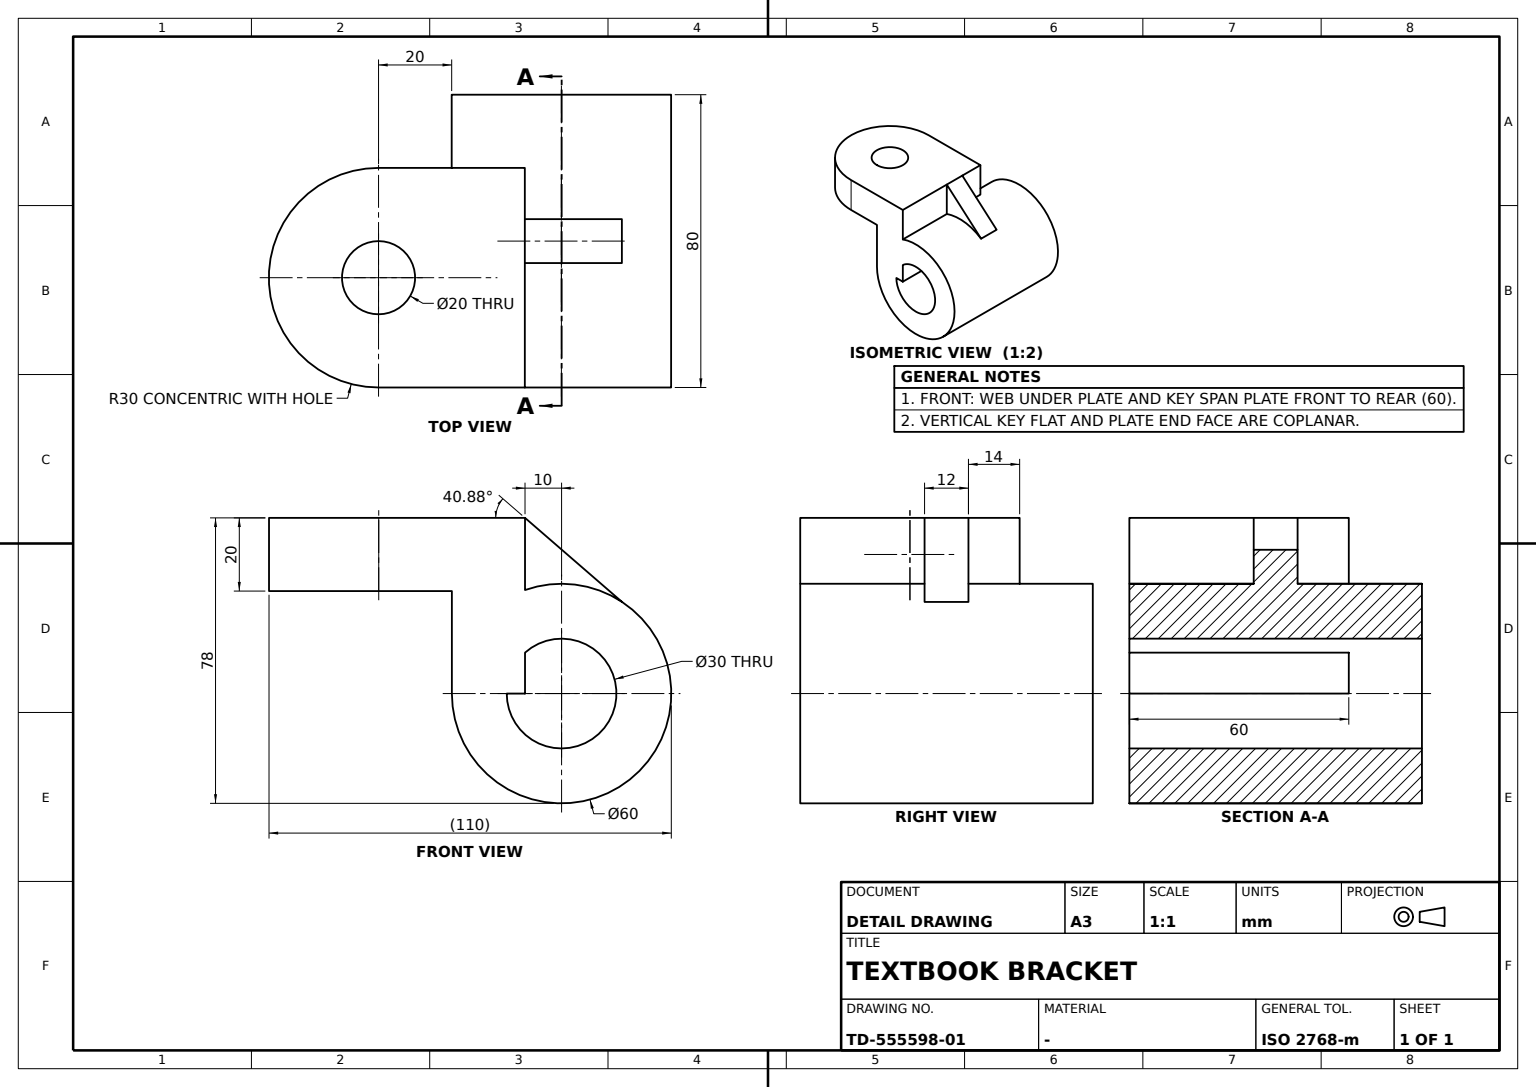
ISO-10303-21;
HEADER;
FILE_DESCRIPTION((''),'2;1');
FILE_NAME('','',(''),(''),'','','');
FILE_SCHEMA(('AUTOMOTIVE_DESIGN'));
ENDSEC;
DATA;
#1=APPLICATION_CONTEXT('');
#2=PRODUCT_CONTEXT('',#1,'mechanical');
#3=PRODUCT('','','',(#2));
#4=PRODUCT_DEFINITION_FORMATION('','',#3);
#5=PRODUCT_DEFINITION_CONTEXT('',#1,'design');
#6=PRODUCT_DEFINITION('','',#4,#5);
#7=PRODUCT_DEFINITION_SHAPE('','',#6);
#8=(LENGTH_UNIT()NAMED_UNIT(*)SI_UNIT(.MILLI.,.METRE.));
#9=(NAMED_UNIT(*)PLANE_ANGLE_UNIT()SI_UNIT($,.RADIAN.));
#10=(NAMED_UNIT(*)SI_UNIT($,.STERADIAN.)SOLID_ANGLE_UNIT());
#11=UNCERTAINTY_MEASURE_WITH_UNIT(LENGTH_MEASURE(0.005),#8,'distance_accuracy_value','');
#12=(GEOMETRIC_REPRESENTATION_CONTEXT(3)GLOBAL_UNCERTAINTY_ASSIGNED_CONTEXT((#11))GLOBAL_UNIT_ASSIGNED_CONTEXT((#8,#9,#10))REPRESENTATION_CONTEXT('',''));
#13=CARTESIAN_POINT('',(-34.,10.,48.));
#14=VERTEX_POINT('',#13);
#15=CARTESIAN_POINT('',(-34.,36.536894,25.030604));
#16=VERTEX_POINT('',#15);
#17=DIRECTION('',(0.,0.756101342,-0.654454553));
#18=VECTOR('',#17,1000.);
#19=LINE('',#13,#18);
#20=EDGE_CURVE('',#14,#16,#19,.T.);
#21=ORIENTED_EDGE('',*,*,#20,.F.);
#22=CARTESIAN_POINT('',(-34.,10.,28.284271));
#23=VERTEX_POINT('',#22);
#24=CARTESIAN_POINT('',(-34.,10.,0.));
#25=DIRECTION('',(0.,0.,-1.));
#26=VECTOR('',#25,1000.);
#27=LINE('',#24,#26);
#28=EDGE_CURVE('',#14,#23,#27,.T.);
#29=ORIENTED_EDGE('',*,*,#28,.T.);
#30=CARTESIAN_POINT('',(-34.,20.,0.));
#31=DIRECTION('',(1.,0.,0.));
#32=AXIS2_PLACEMENT_3D('',#30,#31,#25);
#33=CIRCLE('',#32,30.);
#34=EDGE_CURVE('',#16,#23,#33,.T.);
#35=ORIENTED_EDGE('',*,*,#34,.F.);
#36=EDGE_LOOP('',(#21,#29,#35));
#37=FACE_BOUND('',#36,.T.);
#38=CARTESIAN_POINT('',(-34.,0.,0.));
#39=DIRECTION('',(0.,1.,0.));
#40=AXIS2_PLACEMENT_3D('',#38,#31,#39);
#41=PLANE('',#40);
#42=ADVANCED_FACE('',(#37),#41,.T.);
#43=CARTESIAN_POINT('',(0.,-10.,28.));
#44=VERTEX_POINT('',#43);
#45=CARTESIAN_POINT('',(-60.,-10.,28.));
#46=VERTEX_POINT('',#45);
#47=DIRECTION('',(-1.,0.,0.));
#48=VECTOR('',#47,1000.);
#49=LINE('',#43,#48);
#50=EDGE_CURVE('',#44,#46,#49,.T.);
#51=ORIENTED_EDGE('',*,*,#50,.T.);
#52=CARTESIAN_POINT('',(-60.,-10.,0.));
#53=VERTEX_POINT('',#52);
#54=LINE('',#52,#26);
#55=EDGE_CURVE('',#46,#53,#54,.T.);
#56=ORIENTED_EDGE('',*,*,#55,.T.);
#57=CARTESIAN_POINT('',(0.,-10.,0.));
#58=VERTEX_POINT('',#57);
#59=CARTESIAN_POINT('',(-40.,-10.,0.));
#60=VECTOR('',#31,1000.);
#61=LINE('',#59,#60);
#62=EDGE_CURVE('',#58,#53,#61,.F.);
#63=ORIENTED_EDGE('',*,*,#62,.F.);
#64=DIRECTION('',(0.,0.,1.));
#65=VECTOR('',#64,1000.);
#66=LINE('',#57,#65);
#67=EDGE_CURVE('',#58,#44,#66,.T.);
#68=ORIENTED_EDGE('',*,*,#67,.T.);
#69=EDGE_LOOP('',(#51,#56,#63,#68));
#70=FACE_BOUND('',#69,.T.);
#71=AXIS2_PLACEMENT_3D('',#57,#39,#47);
#72=PLANE('',#71);
#73=ADVANCED_FACE('',(#70),#72,.F.);
#74=CARTESIAN_POINT('',(0.,10.,11.18034));
#75=VERTEX_POINT('',#74);
#76=CARTESIAN_POINT('',(-60.,10.,11.18034));
#77=VERTEX_POINT('',#76);
#78=LINE('',#74,#60);
#79=EDGE_CURVE('',#75,#77,#78,.F.);
#80=ORIENTED_EDGE('',*,*,#79,.F.);
#81=CARTESIAN_POINT('',(0.,10.,0.));
#82=VERTEX_POINT('',#81);
#83=LINE('',#81,#65);
#84=EDGE_CURVE('',#82,#75,#83,.T.);
#85=ORIENTED_EDGE('',*,*,#84,.F.);
#86=CARTESIAN_POINT('',(-60.,10.,0.));
#87=VERTEX_POINT('',#86);
#88=LINE('',#81,#60);
#89=EDGE_CURVE('',#87,#82,#88,.T.);
#90=ORIENTED_EDGE('',*,*,#89,.F.);
#91=LINE('',#86,#26);
#92=EDGE_CURVE('',#77,#87,#91,.T.);
#93=ORIENTED_EDGE('',*,*,#92,.F.);
#94=EDGE_LOOP('',(#80,#85,#90,#93));
#95=FACE_BOUND('',#94,.T.);
#96=AXIS2_PLACEMENT_3D('',#81,#39,#47);
#97=PLANE('',#96);
#98=ADVANCED_FACE('',(#95),#97,.T.);
#99=CARTESIAN_POINT('',(-46.,10.,48.));
#100=VERTEX_POINT('',#99);
#101=CARTESIAN_POINT('',(-60.,10.,48.));
#102=VERTEX_POINT('',#101);
#103=CARTESIAN_POINT('',(0.,10.,48.));
#104=LINE('',#103,#48);
#105=EDGE_CURVE('',#100,#102,#104,.T.);
#106=ORIENTED_EDGE('',*,*,#105,.T.);
#107=CARTESIAN_POINT('',(-60.,-30.,48.));
#108=VERTEX_POINT('',#107);
#109=CARTESIAN_POINT('',(-60.,0.,48.));
#110=DIRECTION('',(0.,-1.,0.));
#111=VECTOR('',#110,1000.);
#112=LINE('',#109,#111);
#113=EDGE_CURVE('',#102,#108,#112,.T.);
#114=ORIENTED_EDGE('',*,*,#113,.T.);
#115=CARTESIAN_POINT('',(0.,-30.,48.));
#116=VERTEX_POINT('',#115);
#117=CARTESIAN_POINT('',(-30.,-30.,48.));
#118=AXIS2_PLACEMENT_3D('',#117,#25,#47);
#119=CIRCLE('',#118,30.);
#120=EDGE_CURVE('',#108,#116,#119,.F.);
#121=ORIENTED_EDGE('',*,*,#120,.T.);
#122=VERTEX_POINT('',#103);
#123=CARTESIAN_POINT('',(0.,0.,48.));
#124=VECTOR('',#39,1000.);
#125=LINE('',#123,#124);
#126=EDGE_CURVE('',#116,#122,#125,.T.);
#127=ORIENTED_EDGE('',*,*,#126,.T.);
#128=EDGE_CURVE('',#122,#14,#104,.T.);
#129=ORIENTED_EDGE('',*,*,#128,.T.);
#130=LINE('',#103,#60);
#131=EDGE_CURVE('',#100,#14,#130,.T.);
#132=ORIENTED_EDGE('',*,*,#131,.F.);
#133=EDGE_LOOP('',(#106,#114,#121,#127,#129,#132));
#134=FACE_BOUND('',#133,.T.);
#135=CARTESIAN_POINT('',(-40.,-30.,48.));
#136=VERTEX_POINT('',#135);
#137=CIRCLE('',#118,10.);
#138=EDGE_CURVE('',#136,#136,#137,.F.);
#139=ORIENTED_EDGE('',*,*,#138,.F.);
#140=EDGE_LOOP('',(#139));
#141=FACE_BOUND('',#140,.T.);
#142=AXIS2_PLACEMENT_3D('',#123,#25,#47);
#143=PLANE('',#142);
#144=ADVANCED_FACE('',(#134,#141),#143,.F.);
#145=CARTESIAN_POINT('',(-80.,20.,-15.));
#146=VERTEX_POINT('',#145);
#147=CARTESIAN_POINT('',(-80.,20.,0.));
#148=AXIS2_PLACEMENT_3D('',#147,#31,#25);
#149=CIRCLE('',#148,15.);
#150=EDGE_CURVE('',#146,#146,#149,.T.);
#151=ORIENTED_EDGE('',*,*,#150,.F.);
#152=EDGE_LOOP('',(#151));
#153=FACE_BOUND('',#152,.T.);
#154=ORIENTED_EDGE('',*,*,#79,.T.);
#155=CARTESIAN_POINT('',(-60.,5.,0.));
#156=VERTEX_POINT('',#155);
#157=CARTESIAN_POINT('',(-60.,20.,0.));
#158=AXIS2_PLACEMENT_3D('',#157,#31,#25);
#159=CIRCLE('',#158,15.);
#160=EDGE_CURVE('',#77,#156,#159,.T.);
#161=ORIENTED_EDGE('',*,*,#160,.T.);
#162=CARTESIAN_POINT('',(0.,5.,0.));
#163=VERTEX_POINT('',#162);
#164=LINE('',#155,#60);
#165=EDGE_CURVE('',#156,#163,#164,.T.);
#166=ORIENTED_EDGE('',*,*,#165,.T.);
#167=CARTESIAN_POINT('',(0.,20.,0.));
#168=AXIS2_PLACEMENT_3D('',#167,#47,#64);
#169=CIRCLE('',#168,15.);
#170=EDGE_CURVE('',#163,#75,#169,.F.);
#171=ORIENTED_EDGE('',*,*,#170,.T.);
#172=EDGE_LOOP('',(#154,#161,#166,#171));
#173=FACE_BOUND('',#172,.T.);
#174=CARTESIAN_POINT('',(-40.,20.,0.));
#175=AXIS2_PLACEMENT_3D('',#174,#31,#39);
#176=CYLINDRICAL_SURFACE('',#175,15.);
#177=ADVANCED_FACE('',(#153,#173),#176,.F.);
#178=CARTESIAN_POINT('',(-60.,-30.,28.));
#179=VERTEX_POINT('',#178);
#180=CARTESIAN_POINT('',(-60.,-30.,38.));
#181=LINE('',#180,#65);
#182=EDGE_CURVE('',#108,#179,#181,.F.);
#183=ORIENTED_EDGE('',*,*,#182,.T.);
#184=CARTESIAN_POINT('',(0.,-30.,28.));
#185=VERTEX_POINT('',#184);
#186=CARTESIAN_POINT('',(-30.,-30.,28.));
#187=AXIS2_PLACEMENT_3D('',#186,#64,#31);
#188=CIRCLE('',#187,30.);
#189=EDGE_CURVE('',#179,#185,#188,.T.);
#190=ORIENTED_EDGE('',*,*,#189,.T.);
#191=CARTESIAN_POINT('',(0.,-30.,38.));
#192=LINE('',#191,#65);
#193=EDGE_CURVE('',#116,#185,#192,.F.);
#194=ORIENTED_EDGE('',*,*,#193,.F.);
#195=ORIENTED_EDGE('',*,*,#120,.F.);
#196=EDGE_LOOP('',(#183,#190,#194,#195));
#197=FACE_BOUND('',#196,.T.);
#198=CARTESIAN_POINT('',(-30.,-30.,38.));
#199=AXIS2_PLACEMENT_3D('',#198,#64,#31);
#200=CYLINDRICAL_SURFACE('',#199,30.);
#201=ADVANCED_FACE('',(#197),#200,.T.);
#202=CARTESIAN_POINT('',(-46.,10.,28.284271));
#203=VERTEX_POINT('',#202);
#204=CARTESIAN_POINT('',(-60.,10.,28.284271));
#205=VERTEX_POINT('',#204);
#206=LINE('',#202,#60);
#207=EDGE_CURVE('',#203,#205,#206,.F.);
#208=ORIENTED_EDGE('',*,*,#207,.T.);
#209=EDGE_CURVE('',#102,#205,#91,.T.);
#210=ORIENTED_EDGE('',*,*,#209,.F.);
#211=ORIENTED_EDGE('',*,*,#105,.F.);
#212=CARTESIAN_POINT('',(-46.,10.,0.));
#213=LINE('',#212,#26);
#214=EDGE_CURVE('',#100,#203,#213,.T.);
#215=ORIENTED_EDGE('',*,*,#214,.T.);
#216=EDGE_LOOP('',(#208,#210,#211,#215));
#217=FACE_BOUND('',#216,.T.);
#218=ADVANCED_FACE('',(#217),#97,.T.);
#219=CARTESIAN_POINT('',(-60.,0.,0.));
#220=LINE('',#219,#124);
#221=EDGE_CURVE('',#156,#87,#220,.T.);
#222=ORIENTED_EDGE('',*,*,#221,.T.);
#223=ORIENTED_EDGE('',*,*,#89,.T.);
#224=CARTESIAN_POINT('',(0.,0.,0.));
#225=LINE('',#224,#124);
#226=EDGE_CURVE('',#163,#82,#225,.T.);
#227=ORIENTED_EDGE('',*,*,#226,.F.);
#228=ORIENTED_EDGE('',*,*,#165,.F.);
#229=EDGE_LOOP('',(#222,#223,#227,#228));
#230=FACE_BOUND('',#229,.T.);
#231=AXIS2_PLACEMENT_3D('',#219,#64,#31);
#232=PLANE('',#231);
#233=ADVANCED_FACE('',(#230),#232,.F.);
#234=ORIENTED_EDGE('',*,*,#189,.F.);
#235=CARTESIAN_POINT('',(-60.,0.,28.));
#236=LINE('',#235,#111);
#237=EDGE_CURVE('',#46,#179,#236,.T.);
#238=ORIENTED_EDGE('',*,*,#237,.F.);
#239=ORIENTED_EDGE('',*,*,#50,.F.);
#240=CARTESIAN_POINT('',(0.,0.,28.));
#241=LINE('',#240,#124);
#242=EDGE_CURVE('',#185,#44,#241,.T.);
#243=ORIENTED_EDGE('',*,*,#242,.F.);
#244=EDGE_LOOP('',(#234,#238,#239,#243));
#245=FACE_BOUND('',#244,.T.);
#246=CARTESIAN_POINT('',(-20.,-30.,28.));
#247=VERTEX_POINT('',#246);
#248=CIRCLE('',#187,10.);
#249=EDGE_CURVE('',#247,#247,#248,.T.);
#250=ORIENTED_EDGE('',*,*,#249,.T.);
#251=EDGE_LOOP('',(#250));
#252=FACE_BOUND('',#251,.T.);
#253=AXIS2_PLACEMENT_3D('',#240,#64,#31);
#254=PLANE('',#253);
#255=ADVANCED_FACE('',(#245,#252),#254,.F.);
#256=ORIENTED_EDGE('',*,*,#28,.F.);
#257=ORIENTED_EDGE('',*,*,#128,.F.);
#258=CARTESIAN_POINT('',(0.,10.,28.284271));
#259=VERTEX_POINT('',#258);
#260=EDGE_CURVE('',#259,#122,#83,.T.);
#261=ORIENTED_EDGE('',*,*,#260,.F.);
#262=LINE('',#258,#60);
#263=EDGE_CURVE('',#259,#23,#262,.F.);
#264=ORIENTED_EDGE('',*,*,#263,.T.);
#265=EDGE_LOOP('',(#256,#257,#261,#264));
#266=FACE_BOUND('',#265,.T.);
#267=ADVANCED_FACE('',(#266),#97,.T.);
#268=ORIENTED_EDGE('',*,*,#170,.F.);
#269=ORIENTED_EDGE('',*,*,#226,.T.);
#270=ORIENTED_EDGE('',*,*,#84,.T.);
#271=EDGE_LOOP('',(#268,#269,#270));
#272=FACE_BOUND('',#271,.T.);
#273=ORIENTED_EDGE('',*,*,#193,.T.);
#274=ORIENTED_EDGE('',*,*,#242,.T.);
#275=ORIENTED_EDGE('',*,*,#67,.F.);
#276=CIRCLE('',#168,30.);
#277=EDGE_CURVE('',#58,#259,#276,.F.);
#278=ORIENTED_EDGE('',*,*,#277,.T.);
#279=ORIENTED_EDGE('',*,*,#260,.T.);
#280=ORIENTED_EDGE('',*,*,#126,.F.);
#281=EDGE_LOOP('',(#273,#274,#275,#278,#279,#280));
#282=FACE_BOUND('',#281,.T.);
#283=AXIS2_PLACEMENT_3D('',#224,#47,#64);
#284=PLANE('',#283);
#285=ADVANCED_FACE('',(#272,#282),#284,.F.);
#286=CARTESIAN_POINT('',(-80.,20.,-30.));
#287=VERTEX_POINT('',#286);
#288=CIRCLE('',#148,30.);
#289=EDGE_CURVE('',#287,#287,#288,.T.);
#290=ORIENTED_EDGE('',*,*,#289,.F.);
#291=EDGE_LOOP('',(#290));
#292=FACE_BOUND('',#291,.T.);
#293=ORIENTED_EDGE('',*,*,#150,.T.);
#294=EDGE_LOOP('',(#293));
#295=FACE_BOUND('',#294,.T.);
#296=CARTESIAN_POINT('',(-80.,0.,0.));
#297=AXIS2_PLACEMENT_3D('',#296,#31,#39);
#298=PLANE('',#297);
#299=ADVANCED_FACE('',(#292,#295),#298,.F.);
#300=CARTESIAN_POINT('',(-46.,36.536894,25.030604));
#301=VERTEX_POINT('',#300);
#302=LINE('',#99,#18);
#303=EDGE_CURVE('',#100,#301,#302,.T.);
#304=ORIENTED_EDGE('',*,*,#303,.T.);
#305=CARTESIAN_POINT('',(-46.,20.,0.));
#306=AXIS2_PLACEMENT_3D('',#305,#31,#25);
#307=CIRCLE('',#306,30.);
#308=EDGE_CURVE('',#301,#203,#307,.T.);
#309=ORIENTED_EDGE('',*,*,#308,.T.);
#310=ORIENTED_EDGE('',*,*,#214,.F.);
#311=EDGE_LOOP('',(#304,#309,#310));
#312=FACE_BOUND('',#311,.T.);
#313=CARTESIAN_POINT('',(-46.,0.,0.));
#314=AXIS2_PLACEMENT_3D('',#313,#31,#39);
#315=PLANE('',#314);
#316=ADVANCED_FACE('',(#312),#315,.F.);
#317=ORIENTED_EDGE('',*,*,#55,.F.);
#318=ORIENTED_EDGE('',*,*,#237,.T.);
#319=ORIENTED_EDGE('',*,*,#182,.F.);
#320=ORIENTED_EDGE('',*,*,#113,.F.);
#321=ORIENTED_EDGE('',*,*,#209,.T.);
#322=CIRCLE('',#158,30.);
#323=EDGE_CURVE('',#205,#53,#322,.T.);
#324=ORIENTED_EDGE('',*,*,#323,.T.);
#325=EDGE_LOOP('',(#317,#318,#319,#320,#321,#324));
#326=FACE_BOUND('',#325,.T.);
#327=AXIS2_PLACEMENT_3D('',#109,#31,#25);
#328=PLANE('',#327);
#329=ADVANCED_FACE('',(#326),#328,.F.);
#330=ORIENTED_EDGE('',*,*,#303,.F.);
#331=ORIENTED_EDGE('',*,*,#131,.T.);
#332=ORIENTED_EDGE('',*,*,#20,.T.);
#333=LINE('',#300,#60);
#334=EDGE_CURVE('',#301,#16,#333,.T.);
#335=ORIENTED_EDGE('',*,*,#334,.F.);
#336=EDGE_LOOP('',(#330,#331,#332,#335));
#337=FACE_BOUND('',#336,.T.);
#338=CARTESIAN_POINT('',(-40.,10.,48.));
#339=DIRECTION('',(0.,0.654454553,0.756101342));
#340=DIRECTION('',(0.,-0.756101342,0.654454553));
#341=AXIS2_PLACEMENT_3D('',#338,#339,#340);
#342=PLANE('',#341);
#343=ADVANCED_FACE('',(#337),#342,.T.);
#344=ORIENTED_EDGE('',*,*,#92,.T.);
#345=ORIENTED_EDGE('',*,*,#221,.F.);
#346=ORIENTED_EDGE('',*,*,#160,.F.);
#347=EDGE_LOOP('',(#344,#345,#346));
#348=FACE_BOUND('',#347,.T.);
#349=ADVANCED_FACE('',(#348),#328,.F.);
#350=ORIENTED_EDGE('',*,*,#263,.F.);
#351=ORIENTED_EDGE('',*,*,#277,.F.);
#352=ORIENTED_EDGE('',*,*,#62,.T.);
#353=ORIENTED_EDGE('',*,*,#323,.F.);
#354=ORIENTED_EDGE('',*,*,#207,.F.);
#355=ORIENTED_EDGE('',*,*,#308,.F.);
#356=ORIENTED_EDGE('',*,*,#334,.T.);
#357=ORIENTED_EDGE('',*,*,#34,.T.);
#358=EDGE_LOOP('',(#350,#351,#352,#353,#354,#355,#356,#357));
#359=FACE_BOUND('',#358,.T.);
#360=ORIENTED_EDGE('',*,*,#289,.T.);
#361=EDGE_LOOP('',(#360));
#362=FACE_BOUND('',#361,.T.);
#363=CYLINDRICAL_SURFACE('',#175,30.);
#364=ADVANCED_FACE('',(#359,#362),#363,.T.);
#365=ORIENTED_EDGE('',*,*,#249,.F.);
#366=EDGE_LOOP('',(#365));
#367=FACE_BOUND('',#366,.T.);
#368=ORIENTED_EDGE('',*,*,#138,.T.);
#369=EDGE_LOOP('',(#368));
#370=FACE_BOUND('',#369,.T.);
#371=CYLINDRICAL_SURFACE('',#199,10.);
#372=ADVANCED_FACE('',(#367,#370),#371,.F.);
#373=CLOSED_SHELL('',(#42,#73,#98,#144,#177,#201,#218,#233,#255,#267,#285,#299,#316,#329,#343,#349,#364,#372));
#374=MANIFOLD_SOLID_BREP('',#373);
#375=ADVANCED_BREP_SHAPE_REPRESENTATION('',(#374),#12);
#376=SHAPE_DEFINITION_REPRESENTATION(#7,#375);
ENDSEC;
END-ISO-10303-21;
